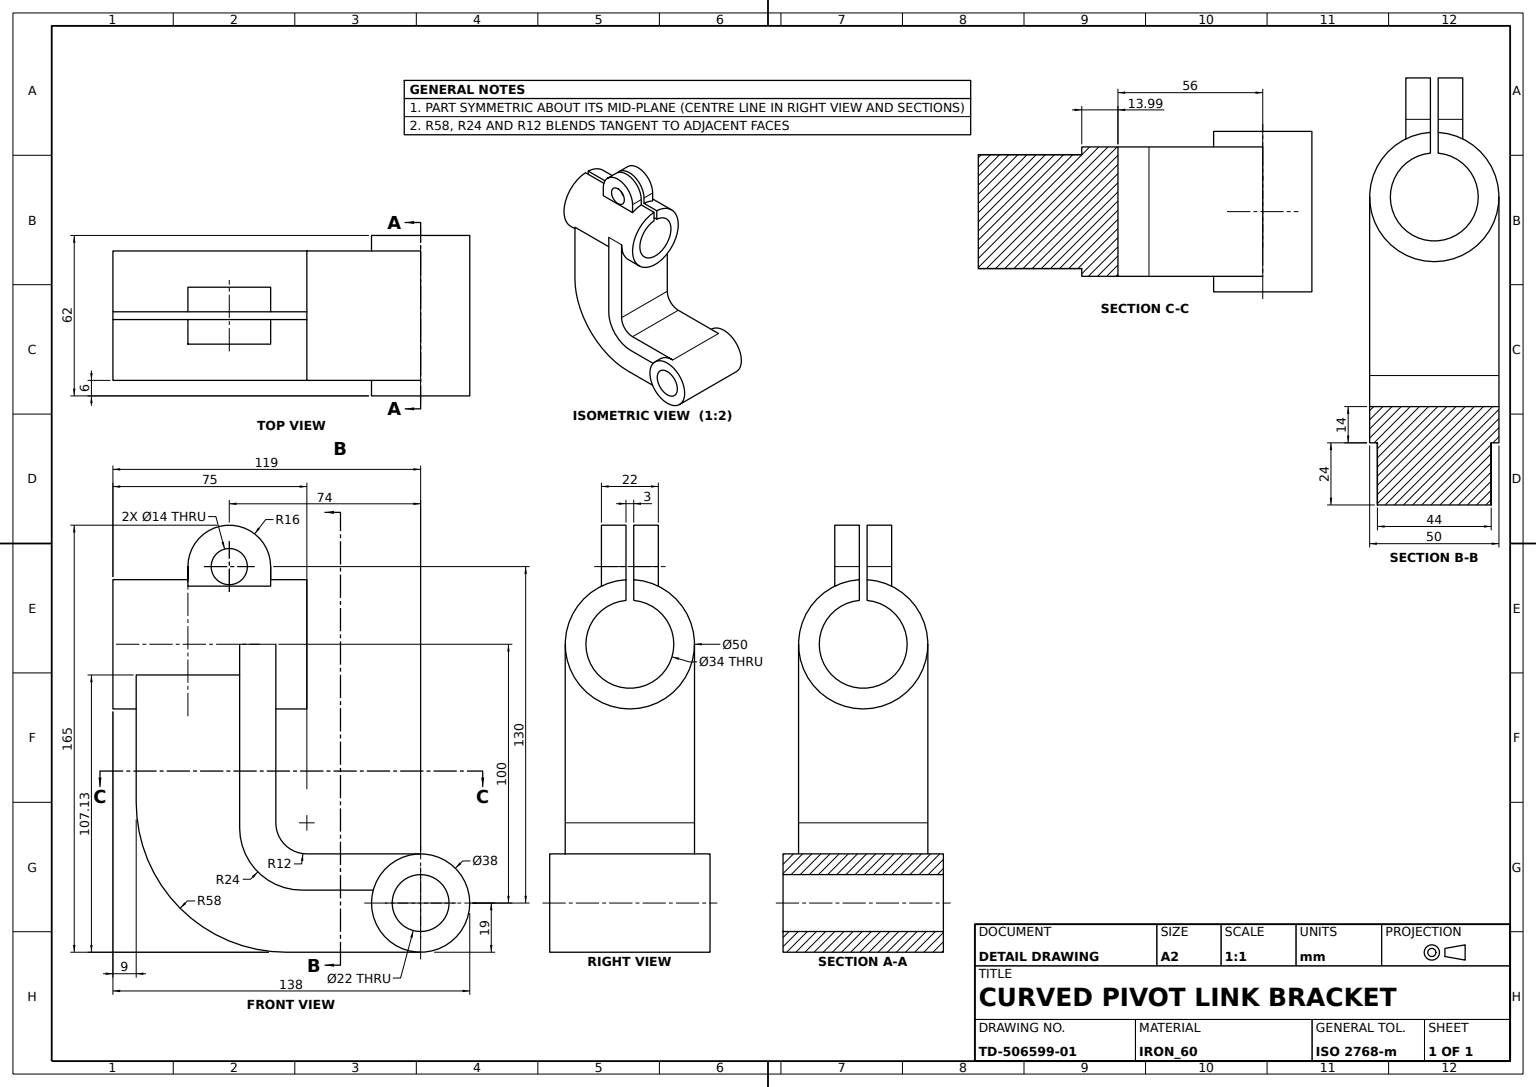
ISO-10303-21;
HEADER;
FILE_DESCRIPTION((''),'2;1');
FILE_NAME('','',(''),(''),'','','');
FILE_SCHEMA(('AUTOMOTIVE_DESIGN'));
ENDSEC;
DATA;
#1=APPLICATION_CONTEXT('');
#2=PRODUCT_CONTEXT('',#1,'mechanical');
#3=PRODUCT('','','',(#2));
#4=PRODUCT_DEFINITION_FORMATION('','',#3);
#5=PRODUCT_DEFINITION_CONTEXT('',#1,'design');
#6=PRODUCT_DEFINITION('','',#4,#5);
#7=PRODUCT_DEFINITION_SHAPE('','',#6);
#8=(LENGTH_UNIT()NAMED_UNIT(*)SI_UNIT(.MILLI.,.METRE.));
#9=(NAMED_UNIT(*)PLANE_ANGLE_UNIT()SI_UNIT($,.RADIAN.));
#10=(NAMED_UNIT(*)SI_UNIT($,.STERADIAN.)SOLID_ANGLE_UNIT());
#11=UNCERTAINTY_MEASURE_WITH_UNIT(LENGTH_MEASURE(0.005),#8,'distance_accuracy_value','');
#12=(GEOMETRIC_REPRESENTATION_CONTEXT(3)GLOBAL_UNCERTAINTY_ASSIGNED_CONTEXT((#11))GLOBAL_UNIT_ASSIGNED_CONTEXT((#8,#9,#10))REPRESENTATION_CONTEXT('',''));
#13=CARTESIAN_POINT('',(-45.990333,-25.,5.));
#14=VERTEX_POINT('',#13);
#15=CARTESIAN_POINT('',(-18.330303,-25.,5.));
#16=VERTEX_POINT('',#15);
#17=CARTESIAN_POINT('',(-69.990333,-25.,5.));
#18=DIRECTION('',(1.,0.,0.));
#19=VECTOR('',#18,1000.);
#20=LINE('',#17,#19);
#21=EDGE_CURVE('',#14,#16,#20,.T.);
#22=ORIENTED_EDGE('',*,*,#21,.F.);
#23=CARTESIAN_POINT('',(-45.990333,-22.,5.));
#24=VERTEX_POINT('',#23);
#25=DIRECTION('',(0.,1.,0.));
#26=VECTOR('',#25,1000.);
#27=LINE('',#13,#26);
#28=EDGE_CURVE('',#14,#24,#27,.T.);
#29=ORIENTED_EDGE('',*,*,#28,.T.);
#30=CARTESIAN_POINT('',(-18.330303,-22.,5.));
#31=VERTEX_POINT('',#30);
#32=CARTESIAN_POINT('',(-69.990333,-22.,5.));
#33=DIRECTION('',(-1.,0.,0.));
#34=VECTOR('',#33,1000.);
#35=LINE('',#32,#34);
#36=EDGE_CURVE('',#31,#24,#35,.T.);
#37=ORIENTED_EDGE('',*,*,#36,.F.);
#38=LINE('',#15,#26);
#39=EDGE_CURVE('',#16,#31,#38,.T.);
#40=ORIENTED_EDGE('',*,*,#39,.F.);
#41=EDGE_LOOP('',(#22,#29,#37,#40));
#42=FACE_BOUND('',#41,.T.);
#43=DIRECTION('',(0.,0.,1.));
#44=AXIS2_PLACEMENT_3D('',#17,#43,#18);
#45=PLANE('',#44);
#46=ADVANCED_FACE('',(#42),#45,.F.);
#47=CARTESIAN_POINT('',(19.,31.,0.));
#48=VERTEX_POINT('',#47);
#49=CARTESIAN_POINT('',(0.,31.,0.));
#50=DIRECTION('',(0.,-1.,0.));
#51=AXIS2_PLACEMENT_3D('',#49,#50,#18);
#52=CIRCLE('',#51,19.);
#53=EDGE_CURVE('',#48,#48,#52,.T.);
#54=ORIENTED_EDGE('',*,*,#53,.T.);
#55=EDGE_LOOP('',(#54));
#56=FACE_BOUND('',#55,.T.);
#57=CARTESIAN_POINT('',(0.,-22.,-19.));
#58=VERTEX_POINT('',#57);
#59=CARTESIAN_POINT('',(0.,-22.,0.));
#60=AXIS2_PLACEMENT_3D('',#59,#25,#18);
#61=CIRCLE('',#60,19.);
#62=EDGE_CURVE('',#58,#31,#61,.T.);
#63=ORIENTED_EDGE('',*,*,#62,.F.);
#64=CARTESIAN_POINT('',(0.,22.,-19.));
#65=VERTEX_POINT('',#64);
#66=LINE('',#57,#26);
#67=EDGE_CURVE('',#58,#65,#66,.T.);
#68=ORIENTED_EDGE('',*,*,#67,.T.);
#69=CARTESIAN_POINT('',(-18.330303,22.,5.));
#70=VERTEX_POINT('',#69);
#71=CARTESIAN_POINT('',(0.,22.,0.));
#72=AXIS2_PLACEMENT_3D('',#71,#25,#18);
#73=CIRCLE('',#72,19.);
#74=EDGE_CURVE('',#65,#70,#73,.T.);
#75=ORIENTED_EDGE('',*,*,#74,.T.);
#76=CARTESIAN_POINT('',(-18.330303,25.,5.));
#77=VERTEX_POINT('',#76);
#78=EDGE_CURVE('',#70,#77,#38,.T.);
#79=ORIENTED_EDGE('',*,*,#78,.T.);
#80=CARTESIAN_POINT('',(0.,25.,19.));
#81=VERTEX_POINT('',#80);
#82=CARTESIAN_POINT('',(0.,25.,0.));
#83=AXIS2_PLACEMENT_3D('',#82,#25,#18);
#84=CIRCLE('',#83,19.);
#85=EDGE_CURVE('',#77,#81,#84,.T.);
#86=ORIENTED_EDGE('',*,*,#85,.T.);
#87=CARTESIAN_POINT('',(0.,-25.,19.));
#88=VERTEX_POINT('',#87);
#89=LINE('',#87,#26);
#90=EDGE_CURVE('',#88,#81,#89,.T.);
#91=ORIENTED_EDGE('',*,*,#90,.F.);
#92=CARTESIAN_POINT('',(0.,-25.,0.));
#93=AXIS2_PLACEMENT_3D('',#92,#25,#18);
#94=CIRCLE('',#93,19.);
#95=EDGE_CURVE('',#16,#88,#94,.T.);
#96=ORIENTED_EDGE('',*,*,#95,.F.);
#97=ORIENTED_EDGE('',*,*,#39,.T.);
#98=EDGE_LOOP('',(#63,#68,#75,#79,#86,#91,#96,#97));
#99=FACE_BOUND('',#98,.T.);
#100=CARTESIAN_POINT('',(19.,-31.,0.));
#101=VERTEX_POINT('',#100);
#102=CARTESIAN_POINT('',(0.,-31.,0.));
#103=AXIS2_PLACEMENT_3D('',#102,#50,#18);
#104=CIRCLE('',#103,19.);
#105=EDGE_CURVE('',#101,#101,#104,.T.);
#106=ORIENTED_EDGE('',*,*,#105,.F.);
#107=EDGE_LOOP('',(#106));
#108=FACE_BOUND('',#107,.T.);
#109=AXIS2_PLACEMENT_3D('',#102,#25,#43);
#110=CYLINDRICAL_SURFACE('',#109,19.);
#111=ADVANCED_FACE('',(#56,#99,#108),#110,.T.);
#112=CARTESIAN_POINT('',(-74.,11.,123.));
#113=VERTEX_POINT('',#112);
#114=CARTESIAN_POINT('',(-74.,11.,130.));
#115=DIRECTION('',(0.,0.,-1.));
#116=AXIS2_PLACEMENT_3D('',#114,#50,#115);
#117=CIRCLE('',#116,7.);
#118=EDGE_CURVE('',#113,#113,#117,.T.);
#119=ORIENTED_EDGE('',*,*,#118,.T.);
#120=EDGE_LOOP('',(#119));
#121=FACE_BOUND('',#120,.T.);
#122=CARTESIAN_POINT('',(-90.,11.,130.));
#123=VERTEX_POINT('',#122);
#124=CARTESIAN_POINT('',(-90.,11.,122.449944));
#125=VERTEX_POINT('',#124);
#126=VECTOR('',#115,1000.);
#127=LINE('',#122,#126);
#128=EDGE_CURVE('',#123,#125,#127,.T.);
#129=ORIENTED_EDGE('',*,*,#128,.F.);
#130=CARTESIAN_POINT('',(-58.,11.,130.));
#131=VERTEX_POINT('',#130);
#132=AXIS2_PLACEMENT_3D('',#114,#50,#18);
#133=CIRCLE('',#132,16.);
#134=EDGE_CURVE('',#131,#123,#133,.T.);
#135=ORIENTED_EDGE('',*,*,#134,.F.);
#136=CARTESIAN_POINT('',(-58.,11.,122.449944));
#137=VERTEX_POINT('',#136);
#138=CARTESIAN_POINT('',(-58.,11.,112.));
#139=VECTOR('',#43,1000.);
#140=LINE('',#138,#139);
#141=EDGE_CURVE('',#137,#131,#140,.T.);
#142=ORIENTED_EDGE('',*,*,#141,.F.);
#143=CARTESIAN_POINT('',(-119.,11.,122.449944));
#144=LINE('',#143,#19);
#145=EDGE_CURVE('',#125,#137,#144,.T.);
#146=ORIENTED_EDGE('',*,*,#145,.F.);
#147=EDGE_LOOP('',(#129,#135,#142,#146));
#148=FACE_BOUND('',#147,.T.);
#149=PLANE('',#116);
#150=ADVANCED_FACE('',(#121,#148),#149,.F.);
#151=CARTESIAN_POINT('',(-119.,-1.5,116.933694));
#152=VERTEX_POINT('',#151);
#153=CARTESIAN_POINT('',(-119.,1.5,116.933694));
#154=VERTEX_POINT('',#153);
#155=CARTESIAN_POINT('',(-119.,0.,100.));
#156=AXIS2_PLACEMENT_3D('',#155,#18,#115);
#157=CIRCLE('',#156,17.);
#158=EDGE_CURVE('',#152,#154,#157,.T.);
#159=ORIENTED_EDGE('',*,*,#158,.F.);
#160=CARTESIAN_POINT('',(-44.,-1.5,116.933694));
#161=VERTEX_POINT('',#160);
#162=LINE('',#160,#34);
#163=EDGE_CURVE('',#152,#161,#162,.F.);
#164=ORIENTED_EDGE('',*,*,#163,.T.);
#165=CARTESIAN_POINT('',(-44.,1.5,116.933694));
#166=VERTEX_POINT('',#165);
#167=CARTESIAN_POINT('',(-44.,0.,100.));
#168=AXIS2_PLACEMENT_3D('',#167,#33,#43);
#169=CIRCLE('',#168,17.);
#170=EDGE_CURVE('',#166,#161,#169,.T.);
#171=ORIENTED_EDGE('',*,*,#170,.F.);
#172=LINE('',#165,#34);
#173=EDGE_CURVE('',#166,#154,#172,.T.);
#174=ORIENTED_EDGE('',*,*,#173,.T.);
#175=EDGE_LOOP('',(#159,#164,#171,#174));
#176=FACE_BOUND('',#175,.T.);
#177=CYLINDRICAL_SURFACE('',#168,17.);
#178=ADVANCED_FACE('',(#176),#177,.F.);
#179=CARTESIAN_POINT('',(0.,31.,-11.));
#180=VERTEX_POINT('',#179);
#181=AXIS2_PLACEMENT_3D('',#49,#50,#115);
#182=CIRCLE('',#181,11.);
#183=EDGE_CURVE('',#180,#180,#182,.T.);
#184=ORIENTED_EDGE('',*,*,#183,.F.);
#185=EDGE_LOOP('',(#184));
#186=FACE_BOUND('',#185,.T.);
#187=CARTESIAN_POINT('',(0.,-31.,11.));
#188=VERTEX_POINT('',#187);
#189=CIRCLE('',#109,11.);
#190=EDGE_CURVE('',#188,#188,#189,.T.);
#191=ORIENTED_EDGE('',*,*,#190,.F.);
#192=EDGE_LOOP('',(#191));
#193=FACE_BOUND('',#192,.T.);
#194=CYLINDRICAL_SURFACE('',#109,11.);
#195=ADVANCED_FACE('',(#186,#193),#194,.F.);
#196=CARTESIAN_POINT('',(-90.,1.5,124.954959));
#197=VERTEX_POINT('',#196);
#198=CARTESIAN_POINT('',(-90.,0.,100.));
#199=AXIS2_PLACEMENT_3D('',#198,#18,#115);
#200=CIRCLE('',#199,25.);
#201=EDGE_CURVE('',#197,#125,#200,.F.);
#202=ORIENTED_EDGE('',*,*,#201,.T.);
#203=ORIENTED_EDGE('',*,*,#145,.T.);
#204=CARTESIAN_POINT('',(-58.,1.5,124.954959));
#205=VERTEX_POINT('',#204);
#206=CARTESIAN_POINT('',(-58.,0.,100.));
#207=AXIS2_PLACEMENT_3D('',#206,#33,#43);
#208=CIRCLE('',#207,25.);
#209=EDGE_CURVE('',#137,#205,#208,.F.);
#210=ORIENTED_EDGE('',*,*,#209,.T.);
#211=CARTESIAN_POINT('',(-44.,1.5,124.954959));
#212=VERTEX_POINT('',#211);
#213=CARTESIAN_POINT('',(-119.,1.5,124.954959));
#214=LINE('',#213,#19);
#215=EDGE_CURVE('',#212,#205,#214,.F.);
#216=ORIENTED_EDGE('',*,*,#215,.F.);
#217=CARTESIAN_POINT('',(-44.,-1.5,124.954959));
#218=VERTEX_POINT('',#217);
#219=AXIS2_PLACEMENT_3D('',#167,#18,#25);
#220=CIRCLE('',#219,25.);
#221=EDGE_CURVE('',#218,#212,#220,.T.);
#222=ORIENTED_EDGE('',*,*,#221,.F.);
#223=CARTESIAN_POINT('',(-58.,-1.5,124.954959));
#224=VERTEX_POINT('',#223);
#225=CARTESIAN_POINT('',(-119.,-1.5,124.954959));
#226=LINE('',#225,#19);
#227=EDGE_CURVE('',#224,#218,#226,.T.);
#228=ORIENTED_EDGE('',*,*,#227,.F.);
#229=CARTESIAN_POINT('',(-58.,-11.,122.449944));
#230=VERTEX_POINT('',#229);
#231=EDGE_CURVE('',#224,#230,#208,.F.);
#232=ORIENTED_EDGE('',*,*,#231,.T.);
#233=CARTESIAN_POINT('',(-90.,-11.,122.449944));
#234=VERTEX_POINT('',#233);
#235=CARTESIAN_POINT('',(-119.,-11.,122.449944));
#236=LINE('',#235,#19);
#237=EDGE_CURVE('',#234,#230,#236,.T.);
#238=ORIENTED_EDGE('',*,*,#237,.F.);
#239=CARTESIAN_POINT('',(-90.,-1.5,124.954959));
#240=VERTEX_POINT('',#239);
#241=EDGE_CURVE('',#234,#240,#200,.F.);
#242=ORIENTED_EDGE('',*,*,#241,.T.);
#243=VERTEX_POINT('',#225);
#244=EDGE_CURVE('',#243,#240,#226,.T.);
#245=ORIENTED_EDGE('',*,*,#244,.F.);
#246=VERTEX_POINT('',#213);
#247=AXIS2_PLACEMENT_3D('',#155,#18,#25);
#248=CIRCLE('',#247,25.);
#249=EDGE_CURVE('',#243,#246,#248,.T.);
#250=ORIENTED_EDGE('',*,*,#249,.T.);
#251=EDGE_CURVE('',#197,#246,#214,.F.);
#252=ORIENTED_EDGE('',*,*,#251,.F.);
#253=EDGE_LOOP('',(#202,#203,#210,#216,#222,#228,#232,#238,#242,#245,#250,#252));
#254=FACE_BOUND('',#253,.T.);
#255=CARTESIAN_POINT('',(-69.990333,22.,88.125658));
#256=VERTEX_POINT('',#255);
#257=CARTESIAN_POINT('',(-69.990333,25.,100.));
#258=VERTEX_POINT('',#257);
#259=CARTESIAN_POINT('',(-69.990333,0.,100.));
#260=AXIS2_PLACEMENT_3D('',#259,#18,#115);
#261=CIRCLE('',#260,25.);
#262=EDGE_CURVE('',#256,#258,#261,.T.);
#263=ORIENTED_EDGE('',*,*,#262,.F.);
#264=CARTESIAN_POINT('',(-110.,22.,88.125658));
#265=VERTEX_POINT('',#264);
#266=CARTESIAN_POINT('',(-119.,22.,88.125658));
#267=LINE('',#266,#19);
#268=EDGE_CURVE('',#256,#265,#267,.F.);
#269=ORIENTED_EDGE('',*,*,#268,.T.);
#270=CARTESIAN_POINT('',(-110.,-22.,88.125658));
#271=VERTEX_POINT('',#270);
#272=CARTESIAN_POINT('',(-110.,0.,100.));
#273=AXIS2_PLACEMENT_3D('',#272,#18,#115);
#274=CIRCLE('',#273,25.);
#275=EDGE_CURVE('',#271,#265,#274,.T.);
#276=ORIENTED_EDGE('',*,*,#275,.F.);
#277=CARTESIAN_POINT('',(-69.990333,-22.,88.125658));
#278=VERTEX_POINT('',#277);
#279=CARTESIAN_POINT('',(-119.,-22.,88.125658));
#280=LINE('',#279,#19);
#281=EDGE_CURVE('',#278,#271,#280,.F.);
#282=ORIENTED_EDGE('',*,*,#281,.F.);
#283=CARTESIAN_POINT('',(-69.990333,-25.,100.));
#284=VERTEX_POINT('',#283);
#285=EDGE_CURVE('',#284,#278,#261,.T.);
#286=ORIENTED_EDGE('',*,*,#285,.F.);
#287=CARTESIAN_POINT('',(-56.,-25.,100.));
#288=VERTEX_POINT('',#287);
#289=LINE('',#287,#34);
#290=EDGE_CURVE('',#288,#284,#289,.T.);
#291=ORIENTED_EDGE('',*,*,#290,.F.);
#292=CARTESIAN_POINT('',(-56.,25.,100.));
#293=VERTEX_POINT('',#292);
#294=CARTESIAN_POINT('',(-56.,0.,100.));
#295=AXIS2_PLACEMENT_3D('',#294,#33,#43);
#296=CIRCLE('',#295,25.);
#297=EDGE_CURVE('',#293,#288,#296,.T.);
#298=ORIENTED_EDGE('',*,*,#297,.F.);
#299=LINE('',#292,#34);
#300=EDGE_CURVE('',#293,#258,#299,.T.);
#301=ORIENTED_EDGE('',*,*,#300,.T.);
#302=EDGE_LOOP('',(#263,#269,#276,#282,#286,#291,#298,#301));
#303=FACE_BOUND('',#302,.T.);
#304=CYLINDRICAL_SURFACE('',#156,25.);
#305=ADVANCED_FACE('',(#254,#303),#304,.T.);
#306=CARTESIAN_POINT('',(-58.,-11.,130.));
#307=VERTEX_POINT('',#306);
#308=CARTESIAN_POINT('',(-58.,-1.5,130.));
#309=VERTEX_POINT('',#308);
#310=LINE('',#306,#26);
#311=EDGE_CURVE('',#307,#309,#310,.T.);
#312=ORIENTED_EDGE('',*,*,#311,.F.);
#313=CARTESIAN_POINT('',(-58.,-11.,112.));
#314=LINE('',#313,#139);
#315=EDGE_CURVE('',#230,#307,#314,.T.);
#316=ORIENTED_EDGE('',*,*,#315,.F.);
#317=ORIENTED_EDGE('',*,*,#231,.F.);
#318=CARTESIAN_POINT('',(-58.,-1.5,112.));
#319=LINE('',#318,#139);
#320=EDGE_CURVE('',#224,#309,#319,.T.);
#321=ORIENTED_EDGE('',*,*,#320,.T.);
#322=EDGE_LOOP('',(#312,#316,#317,#321));
#323=FACE_BOUND('',#322,.T.);
#324=AXIS2_PLACEMENT_3D('',#313,#33,#43);
#325=PLANE('',#324);
#326=ADVANCED_FACE('',(#323),#325,.F.);
#327=ORIENTED_EDGE('',*,*,#190,.T.);
#328=EDGE_LOOP('',(#327));
#329=FACE_BOUND('',#328,.T.);
#330=ORIENTED_EDGE('',*,*,#105,.T.);
#331=EDGE_LOOP('',(#330));
#332=FACE_BOUND('',#331,.T.);
#333=AXIS2_PLACEMENT_3D('',#102,#50,#115);
#334=PLANE('',#333);
#335=ADVANCED_FACE('',(#329,#332),#334,.T.);
#336=ORIENTED_EDGE('',*,*,#221,.T.);
#337=CARTESIAN_POINT('',(-44.,1.5,100.));
#338=LINE('',#337,#139);
#339=EDGE_CURVE('',#166,#212,#338,.T.);
#340=ORIENTED_EDGE('',*,*,#339,.F.);
#341=ORIENTED_EDGE('',*,*,#170,.T.);
#342=CARTESIAN_POINT('',(-44.,-1.5,100.));
#343=LINE('',#342,#126);
#344=EDGE_CURVE('',#218,#161,#343,.T.);
#345=ORIENTED_EDGE('',*,*,#344,.F.);
#346=EDGE_LOOP('',(#336,#340,#341,#345));
#347=FACE_BOUND('',#346,.T.);
#348=AXIS2_PLACEMENT_3D('',#167,#18,#115);
#349=PLANE('',#348);
#350=ADVANCED_FACE('',(#347),#349,.T.);
#351=CARTESIAN_POINT('',(-90.,1.5,130.));
#352=VERTEX_POINT('',#351);
#353=CARTESIAN_POINT('',(-90.,-11.,130.));
#354=LINE('',#353,#26);
#355=EDGE_CURVE('',#352,#123,#354,.T.);
#356=ORIENTED_EDGE('',*,*,#355,.T.);
#357=ORIENTED_EDGE('',*,*,#128,.T.);
#358=ORIENTED_EDGE('',*,*,#201,.F.);
#359=LINE('',#351,#139);
#360=EDGE_CURVE('',#197,#352,#359,.T.);
#361=ORIENTED_EDGE('',*,*,#360,.T.);
#362=EDGE_LOOP('',(#356,#357,#358,#361));
#363=FACE_BOUND('',#362,.T.);
#364=AXIS2_PLACEMENT_3D('',#353,#18,#115);
#365=PLANE('',#364);
#366=ADVANCED_FACE('',(#363),#365,.F.);
#367=CARTESIAN_POINT('',(-74.,1.5,137.));
#368=VERTEX_POINT('',#367);
#369=CARTESIAN_POINT('',(-74.,1.5,130.));
#370=AXIS2_PLACEMENT_3D('',#369,#25,#43);
#371=CIRCLE('',#370,7.);
#372=EDGE_CURVE('',#368,#368,#371,.T.);
#373=ORIENTED_EDGE('',*,*,#372,.T.);
#374=EDGE_LOOP('',(#373));
#375=FACE_BOUND('',#374,.T.);
#376=CARTESIAN_POINT('',(-119.,1.5,100.));
#377=LINE('',#376,#139);
#378=EDGE_CURVE('',#154,#246,#377,.T.);
#379=ORIENTED_EDGE('',*,*,#378,.F.);
#380=ORIENTED_EDGE('',*,*,#173,.F.);
#381=ORIENTED_EDGE('',*,*,#339,.T.);
#382=ORIENTED_EDGE('',*,*,#215,.T.);
#383=CARTESIAN_POINT('',(-58.,1.5,130.));
#384=VERTEX_POINT('',#383);
#385=CARTESIAN_POINT('',(-58.,1.5,112.));
#386=LINE('',#385,#126);
#387=EDGE_CURVE('',#384,#205,#386,.T.);
#388=ORIENTED_EDGE('',*,*,#387,.F.);
#389=CIRCLE('',#370,16.);
#390=EDGE_CURVE('',#352,#384,#389,.T.);
#391=ORIENTED_EDGE('',*,*,#390,.F.);
#392=ORIENTED_EDGE('',*,*,#360,.F.);
#393=ORIENTED_EDGE('',*,*,#251,.T.);
#394=EDGE_LOOP('',(#379,#380,#381,#382,#388,#391,#392,#393));
#395=FACE_BOUND('',#394,.T.);
#396=CARTESIAN_POINT('',(-130.,1.5,100.));
#397=AXIS2_PLACEMENT_3D('',#396,#25,#43);
#398=PLANE('',#397);
#399=ADVANCED_FACE('',(#375,#395),#398,.F.);
#400=ORIENTED_EDGE('',*,*,#118,.F.);
#401=EDGE_LOOP('',(#400));
#402=FACE_BOUND('',#401,.T.);
#403=ORIENTED_EDGE('',*,*,#372,.F.);
#404=EDGE_LOOP('',(#403));
#405=FACE_BOUND('',#404,.T.);
#406=CARTESIAN_POINT('',(-74.,-11.,130.));
#407=AXIS2_PLACEMENT_3D('',#406,#25,#43);
#408=CYLINDRICAL_SURFACE('',#407,7.);
#409=ADVANCED_FACE('',(#402,#405),#408,.F.);
#410=ORIENTED_EDGE('',*,*,#85,.F.);
#411=CARTESIAN_POINT('',(-45.990333,25.,5.));
#412=VERTEX_POINT('',#411);
#413=CARTESIAN_POINT('',(-69.990333,25.,5.));
#414=LINE('',#413,#19);
#415=EDGE_CURVE('',#412,#77,#414,.T.);
#416=ORIENTED_EDGE('',*,*,#415,.F.);
#417=CARTESIAN_POINT('',(-69.990333,25.,29.));
#418=VERTEX_POINT('',#417);
#419=CARTESIAN_POINT('',(-45.990333,25.,29.));
#420=AXIS2_PLACEMENT_3D('',#419,#25,#43);
#421=CIRCLE('',#420,24.);
#422=EDGE_CURVE('',#412,#418,#421,.T.);
#423=ORIENTED_EDGE('',*,*,#422,.T.);
#424=LINE('',#257,#126);
#425=EDGE_CURVE('',#258,#418,#424,.T.);
#426=ORIENTED_EDGE('',*,*,#425,.F.);
#427=ORIENTED_EDGE('',*,*,#300,.F.);
#428=CARTESIAN_POINT('',(-56.,25.,31.));
#429=VERTEX_POINT('',#428);
#430=CARTESIAN_POINT('',(-56.,25.,19.));
#431=LINE('',#430,#139);
#432=EDGE_CURVE('',#429,#293,#431,.T.);
#433=ORIENTED_EDGE('',*,*,#432,.F.);
#434=CARTESIAN_POINT('',(-44.,25.,19.));
#435=VERTEX_POINT('',#434);
#436=CARTESIAN_POINT('',(-44.,25.,31.));
#437=AXIS2_PLACEMENT_3D('',#436,#25,#43);
#438=CIRCLE('',#437,12.);
#439=EDGE_CURVE('',#429,#435,#438,.F.);
#440=ORIENTED_EDGE('',*,*,#439,.T.);
#441=LINE('',#80,#34);
#442=EDGE_CURVE('',#81,#435,#441,.T.);
#443=ORIENTED_EDGE('',*,*,#442,.F.);
#444=EDGE_LOOP('',(#410,#416,#423,#426,#427,#433,#440,#443));
#445=FACE_BOUND('',#444,.T.);
#446=AXIS2_PLACEMENT_3D('',#82,#25,#43);
#447=PLANE('',#446);
#448=ADVANCED_FACE('',(#445),#447,.T.);
#449=ORIENTED_EDGE('',*,*,#442,.T.);
#450=CARTESIAN_POINT('',(-44.,-25.,19.));
#451=VERTEX_POINT('',#450);
#452=LINE('',#450,#26);
#453=EDGE_CURVE('',#435,#451,#452,.F.);
#454=ORIENTED_EDGE('',*,*,#453,.T.);
#455=LINE('',#87,#34);
#456=EDGE_CURVE('',#88,#451,#455,.T.);
#457=ORIENTED_EDGE('',*,*,#456,.F.);
#458=ORIENTED_EDGE('',*,*,#90,.T.);
#459=EDGE_LOOP('',(#449,#454,#457,#458));
#460=FACE_BOUND('',#459,.T.);
#461=AXIS2_PLACEMENT_3D('',#87,#115,#33);
#462=PLANE('',#461);
#463=ADVANCED_FACE('',(#460),#462,.F.);
#464=CARTESIAN_POINT('',(-52.,22.,-19.));
#465=VERTEX_POINT('',#464);
#466=CARTESIAN_POINT('',(-110.,22.,-19.));
#467=LINE('',#466,#19);
#468=EDGE_CURVE('',#465,#65,#467,.T.);
#469=ORIENTED_EDGE('',*,*,#468,.T.);
#470=ORIENTED_EDGE('',*,*,#67,.F.);
#471=CARTESIAN_POINT('',(-52.,-22.,-19.));
#472=VERTEX_POINT('',#471);
#473=CARTESIAN_POINT('',(-110.,-22.,-19.));
#474=LINE('',#473,#19);
#475=EDGE_CURVE('',#472,#58,#474,.T.);
#476=ORIENTED_EDGE('',*,*,#475,.F.);
#477=LINE('',#471,#26);
#478=EDGE_CURVE('',#472,#465,#477,.T.);
#479=ORIENTED_EDGE('',*,*,#478,.T.);
#480=EDGE_LOOP('',(#469,#470,#476,#479));
#481=FACE_BOUND('',#480,.T.);
#482=AXIS2_PLACEMENT_3D('',#473,#43,#18);
#483=PLANE('',#482);
#484=ADVANCED_FACE('',(#481),#483,.F.);
#485=ORIENTED_EDGE('',*,*,#53,.F.);
#486=EDGE_LOOP('',(#485));
#487=FACE_BOUND('',#486,.T.);
#488=ORIENTED_EDGE('',*,*,#183,.T.);
#489=EDGE_LOOP('',(#488));
#490=FACE_BOUND('',#489,.T.);
#491=PLANE('',#181);
#492=ADVANCED_FACE('',(#487,#490),#491,.F.);
#493=ORIENTED_EDGE('',*,*,#262,.T.);
#494=ORIENTED_EDGE('',*,*,#425,.T.);
#495=CARTESIAN_POINT('',(-69.990333,22.,29.));
#496=VERTEX_POINT('',#495);
#497=CARTESIAN_POINT('',(-69.990333,-25.,29.));
#498=LINE('',#497,#26);
#499=EDGE_CURVE('',#418,#496,#498,.F.);
#500=ORIENTED_EDGE('',*,*,#499,.T.);
#501=CARTESIAN_POINT('',(-69.990333,22.,100.));
#502=LINE('',#501,#139);
#503=EDGE_CURVE('',#496,#256,#502,.T.);
#504=ORIENTED_EDGE('',*,*,#503,.T.);
#505=EDGE_LOOP('',(#493,#494,#500,#504));
#506=FACE_BOUND('',#505,.T.);
#507=AXIS2_PLACEMENT_3D('',#283,#18,#115);
#508=PLANE('',#507);
#509=ADVANCED_FACE('',(#506),#508,.F.);
#510=CARTESIAN_POINT('',(-74.,-11.,137.));
#511=VERTEX_POINT('',#510);
#512=CIRCLE('',#407,7.);
#513=EDGE_CURVE('',#511,#511,#512,.T.);
#514=ORIENTED_EDGE('',*,*,#513,.T.);
#515=EDGE_LOOP('',(#514));
#516=FACE_BOUND('',#515,.T.);
#517=VERTEX_POINT('',#353);
#518=LINE('',#353,#126);
#519=EDGE_CURVE('',#517,#234,#518,.T.);
#520=ORIENTED_EDGE('',*,*,#519,.T.);
#521=ORIENTED_EDGE('',*,*,#237,.T.);
#522=ORIENTED_EDGE('',*,*,#315,.T.);
#523=AXIS2_PLACEMENT_3D('',#406,#50,#18);
#524=CIRCLE('',#523,16.);
#525=EDGE_CURVE('',#307,#517,#524,.T.);
#526=ORIENTED_EDGE('',*,*,#525,.T.);
#527=EDGE_LOOP('',(#520,#521,#522,#526));
#528=FACE_BOUND('',#527,.T.);
#529=AXIS2_PLACEMENT_3D('',#406,#50,#115);
#530=PLANE('',#529);
#531=ADVANCED_FACE('',(#516,#528),#530,.T.);
#532=CARTESIAN_POINT('',(-69.990333,-22.,29.));
#533=VERTEX_POINT('',#532);
#534=VERTEX_POINT('',#497);
#535=EDGE_CURVE('',#533,#534,#498,.F.);
#536=ORIENTED_EDGE('',*,*,#535,.F.);
#537=CARTESIAN_POINT('',(-45.990333,-22.,29.));
#538=AXIS2_PLACEMENT_3D('',#537,#25,#43);
#539=CIRCLE('',#538,24.);
#540=EDGE_CURVE('',#24,#533,#539,.T.);
#541=ORIENTED_EDGE('',*,*,#540,.F.);
#542=ORIENTED_EDGE('',*,*,#28,.F.);
#543=CARTESIAN_POINT('',(-45.990333,-25.,29.));
#544=AXIS2_PLACEMENT_3D('',#543,#25,#43);
#545=CIRCLE('',#544,24.);
#546=EDGE_CURVE('',#534,#14,#545,.F.);
#547=ORIENTED_EDGE('',*,*,#546,.F.);
#548=EDGE_LOOP('',(#536,#541,#542,#547));
#549=FACE_BOUND('',#548,.T.);
#550=CYLINDRICAL_SURFACE('',#544,24.);
#551=ADVANCED_FACE('',(#549),#550,.T.);
#552=CARTESIAN_POINT('',(-56.,-25.,31.));
#553=VERTEX_POINT('',#552);
#554=CARTESIAN_POINT('',(-44.,-25.,31.));
#555=AXIS2_PLACEMENT_3D('',#554,#25,#43);
#556=CIRCLE('',#555,12.);
#557=EDGE_CURVE('',#451,#553,#556,.T.);
#558=ORIENTED_EDGE('',*,*,#557,.F.);
#559=ORIENTED_EDGE('',*,*,#453,.F.);
#560=ORIENTED_EDGE('',*,*,#439,.F.);
#561=LINE('',#428,#26);
#562=EDGE_CURVE('',#553,#429,#561,.T.);
#563=ORIENTED_EDGE('',*,*,#562,.F.);
#564=EDGE_LOOP('',(#558,#559,#560,#563));
#565=FACE_BOUND('',#564,.T.);
#566=AXIS2_PLACEMENT_3D('',#554,#50,#115);
#567=CYLINDRICAL_SURFACE('',#566,12.);
#568=ADVANCED_FACE('',(#565),#567,.F.);
#569=ORIENTED_EDGE('',*,*,#355,.F.);
#570=ORIENTED_EDGE('',*,*,#390,.T.);
#571=EDGE_CURVE('',#384,#131,#310,.T.);
#572=ORIENTED_EDGE('',*,*,#571,.T.);
#573=ORIENTED_EDGE('',*,*,#134,.T.);
#574=EDGE_LOOP('',(#569,#570,#572,#573));
#575=FACE_BOUND('',#574,.T.);
#576=CYLINDRICAL_SURFACE('',#407,16.);
#577=ADVANCED_FACE('',(#575),#576,.T.);
#578=ORIENTED_EDGE('',*,*,#249,.F.);
#579=CARTESIAN_POINT('',(-119.,-1.5,100.));
#580=LINE('',#579,#126);
#581=EDGE_CURVE('',#243,#152,#580,.T.);
#582=ORIENTED_EDGE('',*,*,#581,.T.);
#583=ORIENTED_EDGE('',*,*,#158,.T.);
#584=ORIENTED_EDGE('',*,*,#378,.T.);
#585=EDGE_LOOP('',(#578,#582,#583,#584));
#586=FACE_BOUND('',#585,.T.);
#587=PLANE('',#156);
#588=ADVANCED_FACE('',(#586),#587,.F.);
#589=ORIENTED_EDGE('',*,*,#478,.F.);
#590=CARTESIAN_POINT('',(-110.,-22.,39.));
#591=VERTEX_POINT('',#590);
#592=CARTESIAN_POINT('',(-52.,-22.,39.));
#593=AXIS2_PLACEMENT_3D('',#592,#25,#43);
#594=CIRCLE('',#593,58.);
#595=EDGE_CURVE('',#591,#472,#594,.F.);
#596=ORIENTED_EDGE('',*,*,#595,.F.);
#597=CARTESIAN_POINT('',(-110.,22.,39.));
#598=VERTEX_POINT('',#597);
#599=LINE('',#590,#26);
#600=EDGE_CURVE('',#598,#591,#599,.F.);
#601=ORIENTED_EDGE('',*,*,#600,.F.);
#602=CARTESIAN_POINT('',(-52.,22.,39.));
#603=AXIS2_PLACEMENT_3D('',#602,#25,#43);
#604=CIRCLE('',#603,58.);
#605=EDGE_CURVE('',#465,#598,#604,.T.);
#606=ORIENTED_EDGE('',*,*,#605,.F.);
#607=EDGE_LOOP('',(#589,#596,#601,#606));
#608=FACE_BOUND('',#607,.T.);
#609=CYLINDRICAL_SURFACE('',#593,58.);
#610=ADVANCED_FACE('',(#608),#609,.T.);
#611=ORIENTED_EDGE('',*,*,#209,.F.);
#612=ORIENTED_EDGE('',*,*,#141,.T.);
#613=ORIENTED_EDGE('',*,*,#571,.F.);
#614=ORIENTED_EDGE('',*,*,#387,.T.);
#615=EDGE_LOOP('',(#611,#612,#613,#614));
#616=FACE_BOUND('',#615,.T.);
#617=ADVANCED_FACE('',(#616),#325,.F.);
#618=CARTESIAN_POINT('',(-45.990333,22.,5.));
#619=VERTEX_POINT('',#618);
#620=EDGE_CURVE('',#619,#412,#27,.T.);
#621=ORIENTED_EDGE('',*,*,#620,.T.);
#622=ORIENTED_EDGE('',*,*,#415,.T.);
#623=ORIENTED_EDGE('',*,*,#78,.F.);
#624=CARTESIAN_POINT('',(-69.990333,22.,5.));
#625=LINE('',#624,#34);
#626=EDGE_CURVE('',#70,#619,#625,.T.);
#627=ORIENTED_EDGE('',*,*,#626,.T.);
#628=EDGE_LOOP('',(#621,#622,#623,#627));
#629=FACE_BOUND('',#628,.T.);
#630=ADVANCED_FACE('',(#629),#45,.F.);
#631=ORIENTED_EDGE('',*,*,#600,.T.);
#632=CARTESIAN_POINT('',(-110.,-22.,100.));
#633=LINE('',#632,#126);
#634=EDGE_CURVE('',#271,#591,#633,.T.);
#635=ORIENTED_EDGE('',*,*,#634,.F.);
#636=ORIENTED_EDGE('',*,*,#275,.T.);
#637=CARTESIAN_POINT('',(-110.,22.,100.));
#638=LINE('',#637,#126);
#639=EDGE_CURVE('',#265,#598,#638,.T.);
#640=ORIENTED_EDGE('',*,*,#639,.T.);
#641=EDGE_LOOP('',(#631,#635,#636,#640));
#642=FACE_BOUND('',#641,.T.);
#643=AXIS2_PLACEMENT_3D('',#632,#18,#115);
#644=PLANE('',#643);
#645=ADVANCED_FACE('',(#642),#644,.F.);
#646=ORIENTED_EDGE('',*,*,#62,.T.);
#647=ORIENTED_EDGE('',*,*,#36,.T.);
#648=ORIENTED_EDGE('',*,*,#540,.T.);
#649=CARTESIAN_POINT('',(-69.990333,-22.,100.));
#650=LINE('',#649,#139);
#651=EDGE_CURVE('',#533,#278,#650,.T.);
#652=ORIENTED_EDGE('',*,*,#651,.T.);
#653=ORIENTED_EDGE('',*,*,#281,.T.);
#654=ORIENTED_EDGE('',*,*,#634,.T.);
#655=ORIENTED_EDGE('',*,*,#595,.T.);
#656=ORIENTED_EDGE('',*,*,#475,.T.);
#657=EDGE_LOOP('',(#646,#647,#648,#652,#653,#654,#655,#656));
#658=FACE_BOUND('',#657,.T.);
#659=AXIS2_PLACEMENT_3D('',#59,#25,#43);
#660=PLANE('',#659);
#661=ADVANCED_FACE('',(#658),#660,.F.);
#662=ORIENTED_EDGE('',*,*,#557,.T.);
#663=CARTESIAN_POINT('',(-56.,-25.,19.));
#664=LINE('',#663,#139);
#665=EDGE_CURVE('',#553,#288,#664,.T.);
#666=ORIENTED_EDGE('',*,*,#665,.T.);
#667=ORIENTED_EDGE('',*,*,#290,.T.);
#668=LINE('',#283,#126);
#669=EDGE_CURVE('',#284,#534,#668,.T.);
#670=ORIENTED_EDGE('',*,*,#669,.T.);
#671=ORIENTED_EDGE('',*,*,#546,.T.);
#672=ORIENTED_EDGE('',*,*,#21,.T.);
#673=ORIENTED_EDGE('',*,*,#95,.T.);
#674=ORIENTED_EDGE('',*,*,#456,.T.);
#675=EDGE_LOOP('',(#662,#666,#667,#670,#671,#672,#673,#674));
#676=FACE_BOUND('',#675,.T.);
#677=AXIS2_PLACEMENT_3D('',#92,#25,#43);
#678=PLANE('',#677);
#679=ADVANCED_FACE('',(#676),#678,.F.);
#680=CARTESIAN_POINT('',(-90.,-1.5,130.));
#681=VERTEX_POINT('',#680);
#682=LINE('',#680,#126);
#683=EDGE_CURVE('',#681,#240,#682,.T.);
#684=ORIENTED_EDGE('',*,*,#683,.T.);
#685=ORIENTED_EDGE('',*,*,#241,.F.);
#686=ORIENTED_EDGE('',*,*,#519,.F.);
#687=EDGE_CURVE('',#517,#681,#354,.T.);
#688=ORIENTED_EDGE('',*,*,#687,.T.);
#689=EDGE_LOOP('',(#684,#685,#686,#688));
#690=FACE_BOUND('',#689,.T.);
#691=ADVANCED_FACE('',(#690),#365,.F.);
#692=ORIENTED_EDGE('',*,*,#687,.F.);
#693=ORIENTED_EDGE('',*,*,#525,.F.);
#694=ORIENTED_EDGE('',*,*,#311,.T.);
#695=CARTESIAN_POINT('',(-74.,-1.5,130.));
#696=AXIS2_PLACEMENT_3D('',#695,#50,#115);
#697=CIRCLE('',#696,16.);
#698=EDGE_CURVE('',#309,#681,#697,.T.);
#699=ORIENTED_EDGE('',*,*,#698,.T.);
#700=EDGE_LOOP('',(#692,#693,#694,#699));
#701=FACE_BOUND('',#700,.T.);
#702=ADVANCED_FACE('',(#701),#576,.T.);
#703=CARTESIAN_POINT('',(-74.,-1.5,123.));
#704=VERTEX_POINT('',#703);
#705=CIRCLE('',#696,7.);
#706=EDGE_CURVE('',#704,#704,#705,.T.);
#707=ORIENTED_EDGE('',*,*,#706,.F.);
#708=EDGE_LOOP('',(#707));
#709=FACE_BOUND('',#708,.T.);
#710=ORIENTED_EDGE('',*,*,#513,.F.);
#711=EDGE_LOOP('',(#710));
#712=FACE_BOUND('',#711,.T.);
#713=ADVANCED_FACE('',(#709,#712),#408,.F.);
#714=ORIENTED_EDGE('',*,*,#605,.T.);
#715=ORIENTED_EDGE('',*,*,#639,.F.);
#716=ORIENTED_EDGE('',*,*,#268,.F.);
#717=ORIENTED_EDGE('',*,*,#503,.F.);
#718=CARTESIAN_POINT('',(-45.990333,22.,29.));
#719=AXIS2_PLACEMENT_3D('',#718,#25,#43);
#720=CIRCLE('',#719,24.);
#721=EDGE_CURVE('',#496,#619,#720,.F.);
#722=ORIENTED_EDGE('',*,*,#721,.T.);
#723=ORIENTED_EDGE('',*,*,#626,.F.);
#724=ORIENTED_EDGE('',*,*,#74,.F.);
#725=ORIENTED_EDGE('',*,*,#468,.F.);
#726=EDGE_LOOP('',(#714,#715,#716,#717,#722,#723,#724,#725));
#727=FACE_BOUND('',#726,.T.);
#728=AXIS2_PLACEMENT_3D('',#71,#25,#43);
#729=PLANE('',#728);
#730=ADVANCED_FACE('',(#727),#729,.T.);
#731=ORIENTED_EDGE('',*,*,#562,.T.);
#732=ORIENTED_EDGE('',*,*,#432,.T.);
#733=ORIENTED_EDGE('',*,*,#297,.T.);
#734=ORIENTED_EDGE('',*,*,#665,.F.);
#735=EDGE_LOOP('',(#731,#732,#733,#734));
#736=FACE_BOUND('',#735,.T.);
#737=AXIS2_PLACEMENT_3D('',#663,#33,#43);
#738=PLANE('',#737);
#739=ADVANCED_FACE('',(#736),#738,.F.);
#740=ORIENTED_EDGE('',*,*,#721,.F.);
#741=ORIENTED_EDGE('',*,*,#499,.F.);
#742=ORIENTED_EDGE('',*,*,#422,.F.);
#743=ORIENTED_EDGE('',*,*,#620,.F.);
#744=EDGE_LOOP('',(#740,#741,#742,#743));
#745=FACE_BOUND('',#744,.T.);
#746=ADVANCED_FACE('',(#745),#550,.T.);
#747=ORIENTED_EDGE('',*,*,#669,.F.);
#748=ORIENTED_EDGE('',*,*,#285,.T.);
#749=ORIENTED_EDGE('',*,*,#651,.F.);
#750=ORIENTED_EDGE('',*,*,#535,.T.);
#751=EDGE_LOOP('',(#747,#748,#749,#750));
#752=FACE_BOUND('',#751,.T.);
#753=ADVANCED_FACE('',(#752),#508,.F.);
#754=ORIENTED_EDGE('',*,*,#244,.T.);
#755=ORIENTED_EDGE('',*,*,#683,.F.);
#756=ORIENTED_EDGE('',*,*,#698,.F.);
#757=ORIENTED_EDGE('',*,*,#320,.F.);
#758=ORIENTED_EDGE('',*,*,#227,.T.);
#759=ORIENTED_EDGE('',*,*,#344,.T.);
#760=ORIENTED_EDGE('',*,*,#163,.F.);
#761=ORIENTED_EDGE('',*,*,#581,.F.);
#762=EDGE_LOOP('',(#754,#755,#756,#757,#758,#759,#760,#761));
#763=FACE_BOUND('',#762,.T.);
#764=ORIENTED_EDGE('',*,*,#706,.T.);
#765=EDGE_LOOP('',(#764));
#766=FACE_BOUND('',#765,.T.);
#767=CARTESIAN_POINT('',(-130.,-1.5,154.768752));
#768=AXIS2_PLACEMENT_3D('',#767,#50,#115);
#769=PLANE('',#768);
#770=ADVANCED_FACE('',(#763,#766),#769,.F.);
#771=CLOSED_SHELL('',(#46,#111,#150,#178,#195,#305,#326,#335,#350,#366,#399,#409,#448,#463,#484,#492,#509,#531,#551,#568,#577,#588,#610,#617,#630,#645,#661,#679,#691,#702,#713,#730,#739,#746,#753,#770));
#772=MANIFOLD_SOLID_BREP('',#771);
#773=ADVANCED_BREP_SHAPE_REPRESENTATION('',(#772),#12);
#774=SHAPE_DEFINITION_REPRESENTATION(#7,#773);
ENDSEC;
END-ISO-10303-21;
